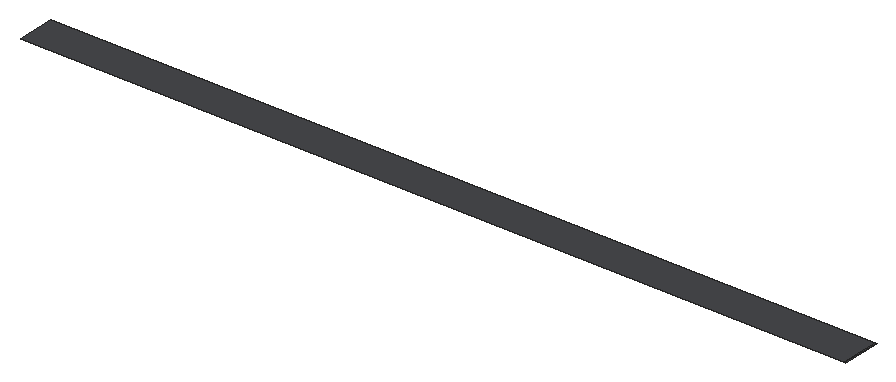
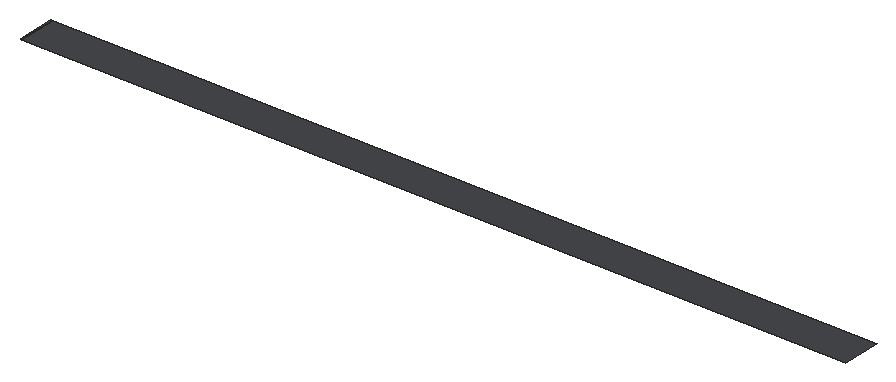
# SketchUp Ruby script. Lengths in inches.
U = 1.inch
M = Sketchup.active_model
def pt(a) = Geom::Point3d.new(a.map { |v| v * U })
def face(e, loops, mat)
  f = e.add_face(loops[0].map { |a| pt(a) })
  loops[1..].each { |l| e.add_face(l.map { |a| pt(a) }).erase! }
  f.material = f.back_material = mat if mat
  f
end
# faces: each face lists its corners as indices into pts; further lists are holes
def faces(e, pts, list, mat = nil) = list.each { |f| face(e, (f[0].is_a?(Array) ? f : [f]).map { |l| l.map { |i| pts[i] } }, mat) }
# xy, xz, yz: faces in a plane at the given z, y or x. An outline is a flat list of corners, or four numbers for a rectangle; further outlines are holes
def ring(l) = l.size == 4 ? [[l[0], l[1]], [l[2], l[1]], [l[2], l[3]], [l[0], l[3]]] : l.each_slice(2).to_a
def flat(e, list, mat, &to3) = list.each { |f| face(e, (f[0].is_a?(Array) ? f : [f]).map { |l| ring(l).map { |u, v| to3.(u, v) } }, mat) }
def xy(e, z, list, mat = nil) = flat(e, list, mat) { |x, y| [x, y, z] }
def xz(e, y, list, mat = nil) = flat(e, list, mat) { |x, z| [x, y, z] }
def yz(e, x, list, mat = nil) = flat(e, list, mat) { |y, z| [x, y, z] }
def lines(e, pts, list) = list.each { |a, b| e.add_line(pt(pts[a]), pt(pts[b])) }
# prism: a flat outline (further loops are holes) pulled along v
def prism(e, loops, v, mat = nil)
  f = face(e, loops, mat); d = Geom::Vector3d.new(v.map { |x| x * U })
  f.pushpull(f.normal.samedirection?(d) ? d.length : -d.length)
end
def box(e, o, s, mat = nil) = prism(e, [[o, [o[0] + s[0], o[1], o[2]], [o[0] + s[0], o[1] + s[1], o[2]], [o[0], o[1] + s[1], o[2]]]], [0, 0, s[2]], mat)
def at(x, y, z, deg = 0) = Geom::Transformation.translation(pt([x, y, z])) * Geom::Transformation.rotation(ORIGIN, Z_AXIS, deg.degrees)
def axes(o, x, y, z) = Geom::Transformation.new([*x, 0, *y, 0, *z, 0, *pt(o).to_a, 1])
def part(name) = M.definitions.add(name)
# library, detail: a bought-in or finely detailed component or shape, given as its bounding box
def library(name, o, s) = part(name).tap { |d| box(d.entities, o, s) }
def detail(e, o, s) = box(e.add_group.entities, o, s)
def put(e, d, t, mat = nil) = e.add_instance(d, t).tap { |i| i.material = mat if mat }
def group(e, t, mat = nil) = e.add_group.tap { |g| g.transformation = t; g.material = mat if mat }.entities
root = M.entities
M.materials.add("1432 AP 8245 TAR ROAD").color = [71, 72, 75]
xy(root,155.79,[[279,95.37,537,107.37],[537,95.37,537.28,107.37]],"1432 AP 8245 TAR ROAD")
p = [[537.28,107.37,155.79],[537.57,107.37,155.8],[537.57,95.37,155.8],[537.28,95.37,155.79]]
faces(root,p,[[0,1,2,3]],"1432 AP 8245 TAR ROAD")
